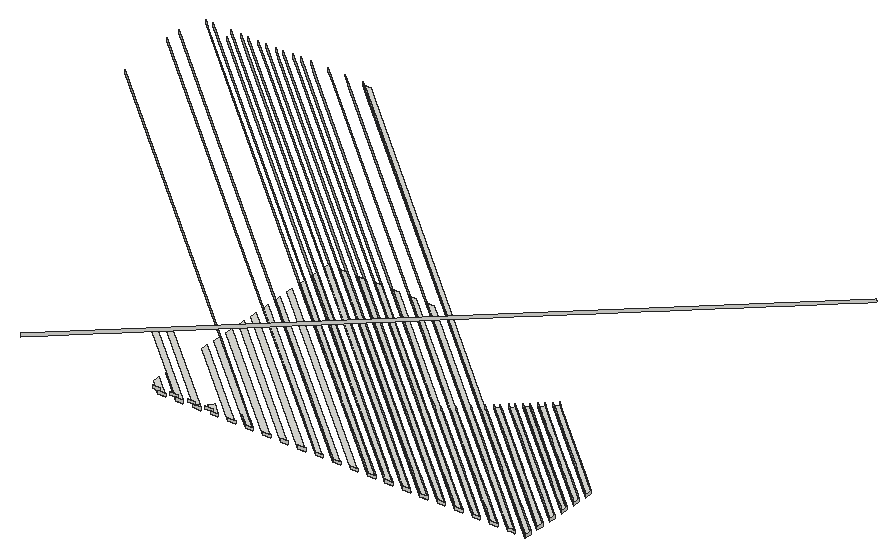
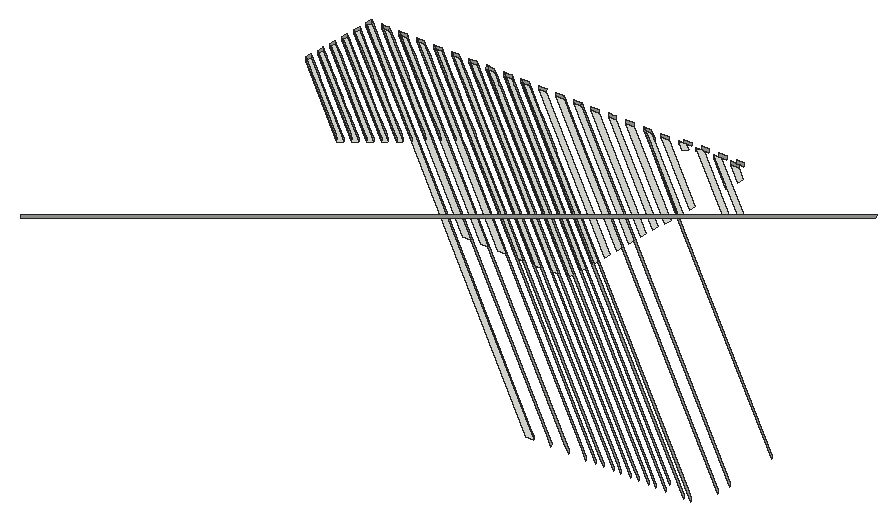
# SketchUp Ruby script. Lengths in inches.
U = 1.inch
M = Sketchup.active_model
def pt(a) = Geom::Point3d.new(a.map { |v| v * U })
def face(e, loops, mat)
  f = e.add_face(loops[0].map { |a| pt(a) })
  loops[1..].each { |l| e.add_face(l.map { |a| pt(a) }).erase! }
  f.material = f.back_material = mat if mat
  f
end
# faces: each face lists its corners as indices into pts; further lists are holes
def faces(e, pts, list, mat = nil) = list.each { |f| face(e, (f[0].is_a?(Array) ? f : [f]).map { |l| l.map { |i| pts[i] } }, mat) }
# xy, xz, yz: faces in a plane at the given z, y or x. An outline is a flat list of corners, or four numbers for a rectangle; further outlines are holes
def ring(l) = l.size == 4 ? [[l[0], l[1]], [l[2], l[1]], [l[2], l[3]], [l[0], l[3]]] : l.each_slice(2).to_a
def flat(e, list, mat, &to3) = list.each { |f| face(e, (f[0].is_a?(Array) ? f : [f]).map { |l| ring(l).map { |u, v| to3.(u, v) } }, mat) }
def xy(e, z, list, mat = nil) = flat(e, list, mat) { |x, y| [x, y, z] }
def xz(e, y, list, mat = nil) = flat(e, list, mat) { |x, z| [x, y, z] }
def yz(e, x, list, mat = nil) = flat(e, list, mat) { |y, z| [x, y, z] }
def lines(e, pts, list) = list.each { |a, b| e.add_line(pt(pts[a]), pt(pts[b])) }
# prism: a flat outline (further loops are holes) pulled along v
def prism(e, loops, v, mat = nil)
  f = face(e, loops, mat); d = Geom::Vector3d.new(v.map { |x| x * U })
  f.pushpull(f.normal.samedirection?(d) ? d.length : -d.length)
end
def box(e, o, s, mat = nil) = prism(e, [[o, [o[0] + s[0], o[1], o[2]], [o[0] + s[0], o[1] + s[1], o[2]], [o[0], o[1] + s[1], o[2]]]], [0, 0, s[2]], mat)
def at(x, y, z, deg = 0) = Geom::Transformation.translation(pt([x, y, z])) * Geom::Transformation.rotation(ORIGIN, Z_AXIS, deg.degrees)
def axes(o, x, y, z) = Geom::Transformation.new([*x, 0, *y, 0, *z, 0, *pt(o).to_a, 1])
def part(name) = M.definitions.add(name)
# library, detail: a bought-in or finely detailed component or shape, given as its bounding box
def library(name, o, s) = part(name).tap { |d| box(d.entities, o, s) }
def detail(e, o, s) = box(e.add_group.entities, o, s)
def put(e, d, t, mat = nil) = e.add_instance(d, t).tap { |i| i.material = mat if mat }
def group(e, t, mat = nil) = e.add_group.tap { |g| g.transformation = t; g.material = mat if mat }.entities
root = M.entities
yz(root,1888.29,[[520.77,107.341,520.796,107.342,520.774,108.369,520.748,108.368]])
yz(root,1888.291,[[507.78,106.881,510.107,106.963,510.084,107.99,507.79,107.909,507.757,107.908],[513.145,107.071,515.433,107.152,515.411,108.179,513.122,108.098],[515.433,107.152,515.472,107.154,515.449,108.181,515.411,108.179]])
yz(root,1888.292,[[497.116,106.503,499.443,106.585,499.421,107.612,497.132,107.531,497.094,107.53],[499.443,106.585,499.469,106.586,499.447,107.613,499.421,107.612],[502.481,106.693,504.421,106.762,504.77,106.774,504.747,107.801,502.459,107.72]])
yz(root,1888.293,[[491.924,106.319,492.427,106.337,494.106,106.396,494.084,107.423,491.901,107.346]])
p = [[1753.93,544.533,108.184],[1814.511,491.919,106.319],[1814.511,491.897,107.346],[1811.832,494.224,107.428],[1801.279,503.388,107.753],[1793.401,510.23,107.996],
  [1762.715,536.881,108.94],[1643.819,640.139,112.601],[1643.819,640.161,111.574],[1753.929,549.831,108.372],[1820.611,491.92,106.319],[1820.611,491.897,107.346],
  [1814.881,496.873,107.522],[1804.329,506.038,107.847],[1801.281,508.684,107.941],[1796.451,512.879,108.089],[1765.765,539.53,109.034],[1643.819,645.437,112.789],
  [1643.819,645.46,111.762],[1784.865,498.606,107.583],[1787.273,496.515,107.509],[1790.321,493.868,107.415],[1792.592,491.895,107.346],[1792.592,491.918,106.319],
  [1785.956,497.682,106.523],[1753.931,525.494,107.509],[1645.138,619.979,110.859],[1645.138,619.956,111.886],[1751.757,527.36,108.603],[1782.442,500.71,107.658],
  [1810.467,511.37,108.036],[1802.589,518.211,108.278],[1800.43,520.087,108.345],[1771.902,544.862,109.223],[1650.696,650.127,112.955],[1646.315,653.932,113.09],
  [1646.315,653.955,112.063],[1650.66,650.181,111.929],[1753.928,560.495,108.75],[1832.888,491.92,106.319],[1832.888,491.898,107.346],[1821.018,502.206,107.711],
  [1815.742,506.788,107.874],[1803.944,519.388,108.32],[1811.821,512.546,108.078],[1822.372,503.383,107.753],[1834.64,492.729,107.375],[1835.597,491.898,107.346],
  [1835.597,491.921,106.319],[1753.928,562.848,108.833],[1649.024,653.955,112.063],[1649.024,653.932,113.09],[1773.257,546.039,109.265],[1836.074,496.783,107.519],
  [1837.69,495.38,107.469],[1840.742,492.73,107.375],[1841.699,491.898,107.346],[1841.699,491.921,106.319],[1753.928,568.148,109.021],[1655.126,653.955,112.063],
  [1655.126,653.933,113.09],[1776.307,548.689,109.359],[1806.995,522.038,108.414],[1814.872,515.197,108.172],[1825.423,506.034,107.847],[1828.509,508.716,107.942],
  [1840.777,498.062,107.564],[1843.829,495.411,107.47],[1847.873,491.899,107.346],[1847.873,491.921,106.319],[1753.935,573.505,109.211],[1661.301,653.955,112.063],
  [1661.301,653.933,113.09],[1779.394,551.371,109.454],[1810.082,524.72,108.509],[1817.959,517.879,108.267],[1757.402,573.505,109.211],[1851.341,491.921,106.319],
  [1851.341,491.899,107.346],[1845.5625,496.917,107.524],[1842.511,499.568,107.618],[1830.243,510.222,107.995],[1819.693,519.385,108.32],[1811.816,526.226,108.5625],
  [1781.128,552.877,109.507],[1671.6,648,112.88],[1664.768,653.933,113.09],[1664.768,653.956,112.063],[1672.223,647.481,111.834],[1831.56,511.367,108.036],
  [1843.828,500.712,107.658],[1846.88,498.062,107.564],[1853.976,491.899,107.346],[1853.976,491.922,106.319],[1760.037,573.505,109.211],[1667.403,653.956,112.063],
  [1667.403,653.933,113.09],[1782.445,554.022,109.548],[1813.133,527.37,108.603],[1821.01,520.529,108.361],[1763.503,573.505,109.211],[1857.441,491.922,106.319],
  [1857.441,491.899,107.346],[1848.612,499.567,107.618],[1845.56,502.217,107.711],[1833.292,512.872,108.089],[1822.742,522.034,108.414],[1814.866,528.875,108.657],
  [1784.178,555.527,109.601],[1675.176,650.193,112.958],[1670.868,653.933,113.09],[1670.868,653.956,112.063],[1675.176,650.215,111.931],[1816.22,530.052,108.698],
  [1824.097,523.211,108.456],[1834.646,514.049,108.131],[1846.915,503.394,107.753],[1849.966,500.744,107.659],[1858.932,492.957,107.383],[1860.15,491.899,107.346],
  [1860.15,491.922,106.319],[1766.212,573.505,109.211],[1673.577,653.956,112.063],[1673.577,653.934,113.09],[1785.532,556.704,109.643],[1769.679,573.506,109.211],
  [1863.618,491.922,106.319],[1863.618,491.9,107.346],[1860.666,494.463,107.437],[1851.7,502.25,107.713],[1848.648,504.9,107.807],[1836.38,515.555,108.184],
  [1825.83,524.717,108.509],[1822.783,527.363,108.603],[1817.954,531.558,108.752],[1787.266,558.21,109.697],[1683.983,647.908,112.877],[1677.045,653.934,113.09],
  [1677.045,653.956,112.063],[1681.352,650.216,111.931],[1819.271,532.702,108.792],[1824.1,528.508,108.644],[1827.147,525.861,108.55],[1837.697,516.7,108.225],
  [1849.965,506.045,107.847],[1853.017,503.394,107.753],[1861.983,495.608,107.477],[1866.252,491.9,107.346],[1866.252,491.922,106.319],[1772.314,573.506,109.211],
  [1679.679,653.957,112.063],[1679.679,653.934,113.09],[1788.583,559.354,109.737],[1775.779,573.506,109.211],[1869.718,491.923,106.319],[1869.718,491.9,107.346],
  [1868.538,492.924,107.382],[1863.715,497.113,107.53],[1854.75,504.899,107.807],[1851.698,507.55,107.901],[1839.429,518.205,108.278],[1828.88,527.367,108.603],
  [1825.833,530.013,108.697],[1821.004,534.207,108.846],[1790.315,560.859,109.79],[1690.639,647.425,112.859],[1683.145,653.934,113.09],[1683.145,653.957,112.063],
  [1688.123,649.634,111.91],[1781.956,573.506,109.211],[1875.894,491.923,106.319],[1875.894,491.9,107.346],[1872.946,494.461,107.436],[1871.626,495.607,107.477],
  [1866.803,499.796,107.626],[1857.838,507.582,107.902],[1854.786,510.233,107.996],[1842.517,520.888,108.373],[1831.968,530.049,108.698],[1828.921,532.695,108.792],
  [1824.092,536.89,108.941],[1793.403,563.542,109.886],[1693.825,650.023,112.952],[1689.321,653.935,113.09],[1689.321,653.957,112.063],[1694.299,649.634,111.91],
  [1788.056,573.507,109.211],[1881.994,491.923,106.319],[1881.994,491.901,107.346],[1875.996,497.11,107.53],[1874.676,498.256,107.571],[1869.853,502.445,107.72],
  [1860.887,510.232,107.996],[1857.835,512.882,108.09],[1845.566,523.538,108.467],[1835.018,532.699,108.792],[1831.971,535.345,108.886],[1827.142,539.539,109.035],
  [1796.453,566.191,109.98],[1699.728,650.195,112.958],[1695.422,653.935,113.09],[1695.422,653.958,112.063],[1700.724,649.352,111.9],[1707.751,648.614,111.874],
  [1701.598,653.958,112.063],[1704.233,653.958,112.063],[1707.751,650.903,111.955],[1796.867,573.507,109.211],[1836.376,539.194,107.995],[1888.293,494.106,106.396],
  [1888.293,492.427,106.337],[1888.293,491.924,106.319],[1888.171,491.924,106.319],[1794.232,573.507,109.211],[1888.171,491.901,107.346],[1879.084,499.793,107.626],
  [1877.764,500.939,107.666],[1872.941,505.128,107.815],[1863.975,512.914,108.091],[1860.923,515.565,108.185],[1848.654,526.221,108.5625],[1838.106,535.382,108.887],
  [1835.059,538.028,108.981],[1830.23,542.222,109.13],[1799.541,568.874,110.075],[1705.637,650.428,112.966],[1701.598,653.935,113.09],[1753.933,504.168,106.753],
  [1768.039,491.917,106.319],[1765.404,491.916,106.319],[1753.933,501.879,106.672],[1789.958,491.918,106.319],[1785.956,495.393,106.442],[1784.746,496.444,106.479],
  [1753.931,523.206,107.428],[1753.929,546.821,108.265],[1817.146,491.919,106.319],[1753.929,552.184,108.455],[1823.32,491.92,106.319],[1820.635,491.92,106.319],
  [1845.164,491.921,106.319],[1839.423,496.908,106.496],[1753.927,571.158,109.128],[1753.927,573.505,109.211],[1839.064,491.921,106.319],[1836.373,494.258,106.402],
  [1753.928,565.86,108.94],[1759.228,491.916,106.319],[1753.933,496.514,106.482],[1753.933,498.867,106.565],[1761.937,491.916,106.319],[1781.349,496.383,106.477],
  [1786.49,491.918,106.319],[1783.781,491.917,106.319],[1753.932,517.841,107.238],[1753.931,520.194,107.321],[1753.931,530.858,107.699],[1798.767,491.918,106.319],
  [1796.058,491.918,106.319],[1753.931,528.505,107.616],[1753.93,536.158,107.887],[1804.869,491.919,106.319],[1802.234,491.919,106.319],[1753.93,533.869,107.806],
  [1753.93,541.521,108.077],[1811.044,491.919,106.319],[1808.334,491.919,106.319],[1753.93,539.168,107.994],[1753.929,557.485,108.643],[1829.422,491.92,106.319],
  [1826.788,491.92,106.319],[1753.929,555.196,108.562],[1759.228,491.893,107.345],[1760.023,491.893,107.345],[1761.937,491.894,107.345],[1765.404,491.894,107.345],
  [1766.125,491.894,107.345],[1768.039,491.894,107.345],[1771.505,491.917,106.319],[1771.505,491.894,107.345],[1772.293,491.894,107.345],[1774.214,491.894,107.345],
  [1774.214,491.917,106.319],[1778.488,573.506,109.211],[1827.1875,531.212,107.712],[1872.427,491.923,106.319],[1777.681,491.917,106.319],[1777.681,491.894,107.345],
  [1778.402,491.895,107.345],[1780.316,491.895,107.345],[1780.316,491.917,106.319],[1784.59,573.507,109.211],[1830.238,533.862,107.806],[1878.529,491.923,106.319],
  [1783.781,491.895,107.346],[1784.577,491.895,107.346],[1786.49,491.895,107.346],[1789.958,491.895,107.346],[1789.004,492.724,107.375],[1785.956,495.371,107.469],
  [1790.765,573.507,109.211],[1833.325,536.544,107.901],[1884.703,491.923,106.319],[1883.349,491.923,106.319],[1790.679,491.895,107.346],[1796.058,491.896,107.346],
  [1796.853,491.896,107.346],[1798.767,491.896,107.346],[1802.955,491.896,107.346],[1804.869,491.896,107.346],[1802.234,491.896,107.346],[1809.154,491.896,107.346],
  [1811.044,491.896,107.346],[1808.334,491.896,107.346],[1815.232,491.897,107.346],[1817.146,491.897,107.346],[1820.635,491.897,107.346],[1821.407,491.897,107.346],
  [1823.32,491.897,107.346],[1829.422,491.898,107.346],[1826.788,491.897,107.346],[1827.509,491.897,107.346],[1872.427,491.9,107.346],[1827.1875,531.189,108.739],
  [1830.234,528.543,108.645],[1840.783,519.382,108.32],[1853.052,508.726,107.942],[1856.104,506.076,107.848],[1865.07,498.289,107.572],[1869.893,494.101,107.424],
  [1871.212,492.955,107.383],[1878.529,491.901,107.346],[1830.238,533.84,108.833],[1833.285,531.194,108.739],[1843.834,522.033,108.414],[1856.103,511.377,108.036],
  [1859.155,508.726,107.942],[1868.121,500.94,107.666],[1872.943,496.751,107.518],[1874.263,495.605,107.477],[1833.683,491.898,107.346],[1884.703,491.901,107.346],
  [1833.325,536.522,108.928],[1836.372,533.876,108.834],[1846.92,524.715,108.509],[1859.19,514.059,108.131],[1862.242,511.408,108.037],[1871.208,503.622,107.761],
  [1876.031,499.433,107.613],[1877.35,498.287,107.572],[1839.064,491.898,107.346],[1836.373,494.236,107.428],[1839.785,491.898,107.346],[1845.164,491.899,107.346],
  [1842.474,494.235,107.428],[1839.423,496.885,107.522],[1851.615,491.899,107.346],[1857.715,491.899,107.346],[1863.891,491.9,107.346],[1869.998,491.9,107.346],
  [1876.168,491.9,107.346],[1882.27,491.901,107.346],[1883.487,491.901,107.346],[1888.293,491.901,107.346],[1888.293,494.084,107.423],[1836.376,539.172,109.022],
  [1839.423,536.526,108.928],[1849.971,527.365,108.603],[1862.24,516.709,108.225],[1865.293,514.059,108.131],[1874.258,506.272,107.855],[1879.081,502.083,107.707],
  [1880.402,500.937,107.666],[1824.106,504.889,107.806],[1813.555,514.053,108.131],[1805.677,520.894,108.374],[1774.99,547.545,109.318],[1656.638,650.331,112.962],
  [1656.638,650.354,111.936],[1665.424,647.999,112.88],[1658.592,653.933,113.09],[1658.592,653.955,112.063],[1666.086,647.447,111.832],[1836.336,499.566,107.617],
  [1827.155,507.539,107.9],[1816.605,516.702,108.225],[1808.727,523.543,108.468],[1778.04,550.195,109.412],[1888.292,497.094,107.53],[1888.292,497.116,106.503],
  [1838.109,540.7,108.048],[1838.109,540.677,109.075],[1841.155,538.031,108.981],[1851.703,528.871,108.656],[1863.973,518.215,108.279],[1867.025,515.564,108.185],
  [1875.991,507.777,107.909],[1880.814,503.589,107.76],[1882.134,502.442,107.719],[1888.292,499.443,106.585],[1888.292,499.469,106.586],[1839.463,541.876,108.09],
  [1868.379,516.741,108.226],[1877.345,508.954,107.95],[1882.168,504.765,107.802],[1883.489,503.618,107.761],[1888.292,499.447,107.613],[1839.463,541.854,109.117],
  [1842.51,539.208,109.023],[1853.057,530.048,108.698],[1865.327,519.391,108.32],[1888.292,502.481,106.693],[1888.292,502.459,107.72],[1885.223,505.124,107.815],
  [1883.902,506.271,107.855],[1879.079,510.46,108.004],[1870.113,518.247,108.28],[1867.061,520.897,108.374],[1854.791,531.554,108.752],[1844.243,540.714,109.076],
  [1841.197,543.36,109.17],[1841.197,543.382,108.143],[1888.292,504.421,106.762],[1888.292,504.77,106.774],[1842.514,544.527,108.184],[1888.292,504.747,107.801],
  [1842.514,544.504,109.211],[1845.561,541.858,109.117],[1856.108,532.698,108.792],[1868.378,522.042,108.414],[1871.43,519.391,108.32],[1880.396,511.605,108.044],
  [1885.219,507.416,107.896],[1886.54,506.269,107.855],[1888.291,507.78,106.881],[1888.291,510.107,106.963],[1845.601,547.208,108.279],[1844.247,546.032,108.237],
  [1888.291,507.757,107.908],[1888.273,507.774,107.908],[1886.952,508.921,107.949],[1882.128,513.11,108.098],[1873.163,520.896,108.374],[1870.111,523.547,108.468],
  [1857.84,534.204,108.845],[1847.293,543.363,109.17],[1844.247,546.009,109.264],[1845.601,547.186,109.306],[1848.646,544.539,109.212],[1859.189,535.376,108.887],
  [1871.456,524.716,108.509],[1874.507,522.064,108.415],[1883.469,514.275,108.139],[1888.291,510.084,107.99],[1888.291,510.133,106.964],[1888.291,512.96,107.065],
  [1888.504,512.96,107.065],[1888.291,513.145,107.071],[1847.335,548.714,108.332],[1888.291,515.433,107.152],[1848.652,549.859,108.373],[1879.071,521.114,108.411],
  [1877.752,522.257,108.452],[1874.922,524.71,108.539],[1871.831,527.39,108.634],[1870.096,528.893,108.687],[1868.777,530.036,108.727],[1867.042,531.541,108.781],
  [1865.686,532.716,108.822],[1863.951,534.219,108.876],[1862.633,535.362,108.916],[1857.807,539.546,109.065],[1856.488,540.689,109.105],[1854.753,542.193,109.158],
  [1853.397,543.368,109.2],[1851.662,544.872,109.253],[1848.608,547.519,109.347],[1847.252,548.695,109.389],[1847.252,548.718,108.332],[1888.291,513.122,108.098],
  [1888.291,513.122,108.128],[1886.95,514.284,108.169],[1883.897,516.93,108.263],[1882.161,518.435,108.316],[1880.806,519.61,108.358],[1886.534,516.937,108.233],
  [1888.291,515.411,108.179],[1848.652,549.836,109.4],[1851.698,547.19,109.306],[1862.245,538.031,108.981],[1874.516,527.374,108.603],[1877.568,524.723,108.509],
  [1811.816,579.539,110.453],[1813.133,580.683,110.493],[1814.866,582.188,110.547],[1816.22,583.365,110.588],[1817.954,584.871,110.642],[1819.271,586.015,110.682],
  [1821.004,587.521,110.736],[1822.358,588.697,110.777],[1824.092,590.203,110.831],[1825.409,591.348,110.871],[1827.141,592.853,110.925],[1828.496,594.03,110.966],
  [1830.229,595.536,111.02],[1831.547,596.68,111.06],[1833.279,598.185,111.114],[1834.633,599.362,111.155],[1836.367,600.868,111.209],[1837.684,602.012,111.249],
  [1839.417,603.517,111.303],[1840.771,604.694,111.345],[1842.505,606.2,111.398],[1843.822,607.345,111.438],[1845.554,608.85,111.492],[1846.909,610.026,111.534],
  [1848.642,611.532,111.587],[1849.96,612.677,111.628],[1851.692,614.182,111.681],[1853.046,615.359,111.723],[1854.78,616.865,111.776],[1856.097,618.009,111.817],
  [1857.83,619.514,111.87],[1859.184,620.691,111.912],[1860.918,622.197,111.965],[1862.235,623.341,112.006],[1863.967,624.847,112.059],[1865.322,626.023,112.101],
  [1867.055,627.529,112.154],[1868.373,628.674,112.195],[1870.105,630.179,112.248],[1871.46,631.355,112.29],[1873.193,632.862,112.343],[1874.51,634.006,112.384],
  [1875.932,635.241,112.428],[1877.287,636.418,112.469],[1879.02,637.924,112.523],[1880.337,639.068,112.563],[1882.07,640.574,112.617],[1883.424,641.75,112.658],
  [1885.158,643.256,112.712],[1886.475,644.401,112.752],[1888.208,645.906,112.806],[1888.281,645.969,112.808],[1888.281,645.946,113.864],[1710.929,491.867,108.402],
  [1710.929,491.891,107.345],[1711.88,492.716,107.375],[1713.613,494.222,107.428],[1714.93,495.367,107.469],[1716.663,496.872,107.522],[1718.017,498.048,107.564],
  [1719.751,499.555,107.617],[1721.068,500.699,107.658],[1722.801,502.204,107.711],[1724.155,503.381,107.753],[1725.889,504.887,107.806],[1727.206,506.031,107.847],
  [1728.938,507.536,107.9],[1730.293,508.713,107.942],[1732.026,510.219,107.995],[1733.344,511.363,108.036],[1735.076,512.869,108.089],[1736.43,514.045,108.131],
  [1738.164,515.551,108.184],[1739.481,516.696,108.225],[1741.214,518.201,108.278],[1742.568,519.378,108.32],[1744.302,520.884,108.373],[1745.619,522.028,108.414],
  [1747.351,523.533,108.467],[1748.706,524.71,108.509],[1750.439,526.216,108.562],[1753.489,528.866,108.656],[1754.844,530.042,108.698],[1756.577,531.548,108.751],
  [1757.894,532.693,108.792],[1759.627,534.198,108.845],[1760.981,535.374,108.887],[1764.032,538.025,108.981],[1767.119,540.707,109.076],[1768.852,542.213,109.129],
  [1770.17,543.357,109.17],[1791.67,562.036,109.832],[1794.72,564.686,109.926],[1797.807,567.368,110.021],[1800.858,570.019,110.115],[1802.591,571.524,110.169],
  [1803.945,572.7,110.21],[1805.679,574.206,110.264],[1806.996,575.351,110.304],[1808.728,576.856,110.358],[1810.083,578.033,110.399],[1773.253,492.728,107.375],
  [1772.297,491.897,107.346],[1760.023,491.87,108.402],[1760.023,491.893,107.375],[1757.314,491.893,107.345],[1757.314,491.893,107.375],[1757.314,491.87,108.402],
  [1766.125,491.893,107.375],[1763.491,491.894,107.345],[1763.491,491.893,107.375],[1763.491,491.87,108.402],[1766.125,491.871,108.402],[1769.591,491.893,107.375],
  [1769.591,491.871,108.402],[1772.293,491.871,108.402],[1769.591,491.894,107.345],[1776.304,495.378,107.469],[1774.987,494.234,107.428],[1775.767,491.871,108.402],
  [1778.402,491.871,108.402],[1778.402,491.894,107.375],[1775.767,491.894,107.345],[1775.767,491.894,107.375],[1888.291,518.443,107.259],[1888.291,518.421,108.286],
  [1888.266,518.442,108.287],[1879.3,526.229,108.563],[1876.248,528.879,108.657],[1863.977,539.537,109.035],[1853.431,548.696,109.359],[1850.385,551.341,109.453],
  [1850.385,551.364,108.426],[1851.739,552.54,108.468],[1888.29,520.796,107.342],[1888.29,520.77,107.341],[1888.29,520.748,108.368],[1888.291,518.463,108.287],
  [1851.739,552.518,109.495],[1854.785,549.872,109.401],[1865.331,540.713,109.076],[1877.602,530.056,108.698],[1880.655,527.405,108.604],[1888.29,520.774,108.369]]
faces(root,p,[[0,1,2,3,4,5,6,7,8],[9,10,11,12,13,14,15,16,17,18],[19,20,21,22,23,24,25,26,27,28,29],[30,31,32,33,34,35,36,37,38,39,40,41,42],[43,44,45,46,47,48,49,50,51,52],[53,54,55,56,57,58,59,60,61,62,63,64],[65,66,67,68,69,70,71,72,73,74,75],[76,77,78,79,80,81,82,83,84,85,86,87,88],
  [89,90,91,92,93,94,95,96,97,98,99],[100,101,102,103,104,105,106,107,108,109,110,111,112],[113,114,115,116,117,118,119,120,121,122,123,124],[125,126,127,128,129,130,131,132,133,134,135,136,137,138,139],[140,141,142,143,144,145,146,147,148,149,150,151,152],[153,154,155,156,157,158,159,160,161,162,163,164,165,166,167,168],[169,170,171,172,173,174,175,176,177,178,179,180,181,182,183,184,185],[186,187,188,189,190,191,192,193,194,195,196,197,198,199,200,201,202],
  [203,204,205,206,207,208,209,210,211,212,213],[213,212,214,215,216,217,218,219,220,221,222,223,224,225,226,204,203],[227,228,229,230],[24,23,231,232,233,234,25],[235,236,1,0],[49,48,39,38],[237,238,239,10,9],[70,69,240,241,242,243],
  [58,57,244,245,246],[247,248,249,250],[251,252,253,254,255],[256,257,258,259],[260,261,262,263],[264,265,266,267],[268,269,270,271],[94,93,77,76],
  [272,273,274,250,247],[121,120,101,100],[275,276,277,228,229],[149,148,126,125],[278,279,280,281,282],[283,284,285,154,153],[286,287,288,289,290],[291,292,293,170,169],
  [294,295,296,252,253],[232,231,297,298,299],[300,301,302,303,187,186],[297,304,22,23,231],[305,306,307,257,258],[308,309,261,262,310],[311,312,265,266,313],[314,315,236,1,2],
  [10,11,316,239],[317,318,238,239,316],[319,269,270,320,321],[322,285,284,323,324,325,326,327,328,329,330],[331,293,292,332,333,334,335,336,337,338,339],[48,39,40,340,47],[341,302,301,342,343,344,345,346,347,348,349],[244,350,351,245],
  [350,352,56,57,244],[240,353,354,355,241],[68,69,240,353],[78,356,92,93,77],[119,120,101,102,357],[358,147,148,126,127],[154,155,359,322,285],[171,360,331,293,170],
  [341,302,303,187,188,361,362],[214,363,211,212],[364,209,208,365,366,367,368,369,370,371,372],[351,373,374,375,376,377,378,246,245],[379,380,381,382,242,241,355,383,384,385,386,387],[388,389,390,391,392,393,394,395,396,397,398],[390,389,399,400,401],[402,403,404,405,406,400,401,407,408,409,410],
  [411,412,413,414,415,416,417,418,419,420,421],[421,411,422,423,424],[425,423,424,426,427,428,429,430,431,432,433],[434,435,436,437],[434,438,439,440,441,442,443,444,445,446,437],[435,436,447,448,449,450,451,452,453],[454,436,435],[455,456,457],
  [458,457,459,460],[461,462,463,464,465,466,467,468,469,470,471,472,473,474,475,476,477,478,457,479,480,481,482,483,484],[485,486,459,460,487,488,489,490,491],[492,493,494,495,496,497,498,499,500,501,502,503,504,505,506,507,508,509,510,511,512,513,514,515,516,517,518,519,520,521,522,523,524,525,526,527,528,529,530,531,532,533,534,535,536,537,538,539,540,541,542,543,544,545,546,547,548,549,550,551,552,553,554,555,556,557,558,559,560,561,562,563,564,565,566,567,568,569,570,571,572,28,573,574,575,576,577,578,6,579,16,580,581,582,33,52,376,61,387,73,84,97,108,124,135,152,164,583,181,584,198,585,224,586,587,588,589,590,591,592],[277,565,564,275,276],[593,567,566,279,280,594],[595,596,273,272,597,598,599],[600,276,275,601,602,603,604],
  [605,606,607,280,279,608],[281,593,594,280],[289,609,610,287,288],[611,612,613,288,287,614,615],[616,617,618,619,620,621,622,623,624],[616,624,625,626,627],[616,627,628,629,617],[630,631,632,633,634,635,626,625]])
